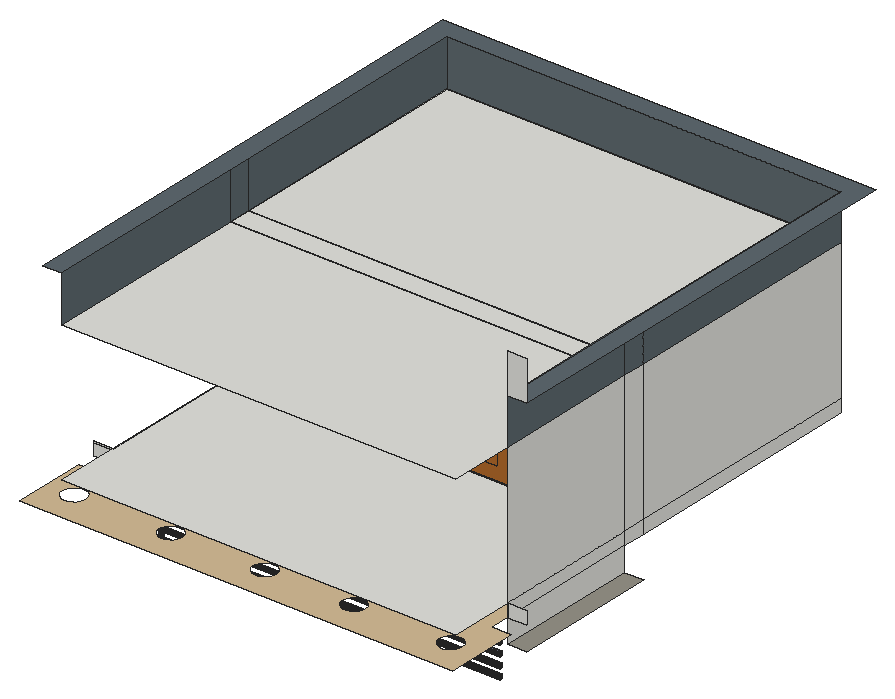
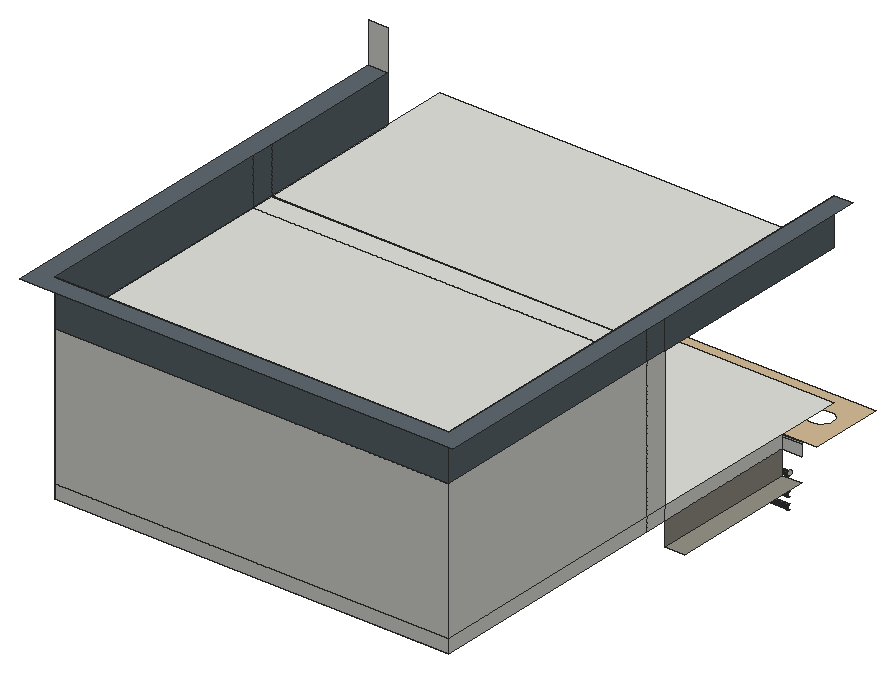
# SketchUp Ruby script. Lengths in inches.
U = 1.inch
M = Sketchup.active_model
def pt(a) = Geom::Point3d.new(a.map { |v| v * U })
def face(e, loops, mat)
  f = e.add_face(loops[0].map { |a| pt(a) })
  loops[1..].each { |l| e.add_face(l.map { |a| pt(a) }).erase! }
  f.material = f.back_material = mat if mat
  f
end
# faces: each face lists its corners as indices into pts; further lists are holes
def faces(e, pts, list, mat = nil) = list.each { |f| face(e, (f[0].is_a?(Array) ? f : [f]).map { |l| l.map { |i| pts[i] } }, mat) }
# xy, xz, yz: faces in a plane at the given z, y or x. An outline is a flat list of corners, or four numbers for a rectangle; further outlines are holes
def ring(l) = l.size == 4 ? [[l[0], l[1]], [l[2], l[1]], [l[2], l[3]], [l[0], l[3]]] : l.each_slice(2).to_a
def flat(e, list, mat, &to3) = list.each { |f| face(e, (f[0].is_a?(Array) ? f : [f]).map { |l| ring(l).map { |u, v| to3.(u, v) } }, mat) }
def xy(e, z, list, mat = nil) = flat(e, list, mat) { |x, y| [x, y, z] }
def xz(e, y, list, mat = nil) = flat(e, list, mat) { |x, z| [x, y, z] }
def yz(e, x, list, mat = nil) = flat(e, list, mat) { |y, z| [x, y, z] }
def lines(e, pts, list) = list.each { |a, b| e.add_line(pt(pts[a]), pt(pts[b])) }
# prism: a flat outline (further loops are holes) pulled along v
def prism(e, loops, v, mat = nil)
  f = face(e, loops, mat); d = Geom::Vector3d.new(v.map { |x| x * U })
  f.pushpull(f.normal.samedirection?(d) ? d.length : -d.length)
end
def box(e, o, s, mat = nil) = prism(e, [[o, [o[0] + s[0], o[1], o[2]], [o[0] + s[0], o[1] + s[1], o[2]], [o[0], o[1] + s[1], o[2]]]], [0, 0, s[2]], mat)
def at(x, y, z, deg = 0) = Geom::Transformation.translation(pt([x, y, z])) * Geom::Transformation.rotation(ORIGIN, Z_AXIS, deg.degrees)
def axes(o, x, y, z) = Geom::Transformation.new([*x, 0, *y, 0, *z, 0, *pt(o).to_a, 1])
def part(name) = M.definitions.add(name)
# library, detail: a bought-in or finely detailed component or shape, given as its bounding box
def library(name, o, s) = part(name).tap { |d| box(d.entities, o, s) }
def detail(e, o, s) = box(e.add_group.entities, o, s)
def put(e, d, t, mat = nil) = e.add_instance(d, t).tap { |i| i.material = mat if mat }
def group(e, t, mat = nil) = e.add_group.tap { |g| g.transformation = t; g.material = mat if mat }.entities
root = M.entities
M.materials.add("[Blinds Cloth Horizontal]").color = [192, 163, 85]
M.materials.add("[Formica Beige]").color = [211, 187, 149]
M.materials.add("[Formica Graystone]").color = [149, 146, 135]
M.materials.add("[Formica Laminate Dark]").color = [50, 53, 60]
M.materials.add("[Formica Speckled Grey]").color = [94, 105, 111]
M.materials.add("[Metal Steel Textured]").color = [106, 110, 123]
M.materials.add("[Wood Bamboo]").color = [177, 105, 43]
M.materials.add("[Wood Cherry Original]").color = [152, 86, 42]
xy(root,38.97,[[48.11,54.44,47.99,54.46,47.89,54.5,47.8,54.57,47.73,54.66,47.68,54.77,47.67,54.88,47.68,54.99,47.73,55.1,47.8,55.19,47.89,55.26,47.99,55.3,48.11,55.32,48.22,55.3,48.33,55.26,48.42,55.19,48.49,55.1,48.53,54.99,48.54,54.88,48.53,54.77,48.49,54.66,48.42,54.57,48.33,54.5,48.22,54.46]])
xy(root,39.16,[[51.04,54.44,50.93,54.46,50.83,54.5,50.74,54.57,50.67,54.66,50.62,54.77,50.61,54.88,50.62,54.99,50.67,55.1,50.74,55.19,50.83,55.26,50.93,55.3,51.04,55.32,51.16,55.3,51.26,55.26,51.35,55.19,51.42,55.1,51.47,54.99,51.48,54.88,51.47,54.77,51.42,54.66,51.35,54.57,51.26,54.5,51.16,54.46]])
xy(root,39.53,[[68.17,54.44,68.06,54.46,67.95,54.5,67.86,54.57,67.79,54.66,67.75,54.77,67.73,54.88,67.75,54.99,67.79,55.1,67.86,55.19,67.95,55.26,68.06,55.3,68.17,55.32,68.28,55.3,68.39,55.26,68.48,55.19,68.55,55.1,68.59,54.99,68.61,54.88,68.59,54.77,68.55,54.66,68.48,54.57,68.39,54.5,68.28,54.46]])
xy(root,39.72,[[71.42,54.44,71.31,54.46,71.2,54.5,71.11,54.57,71.04,54.66,71,54.77,70.98,54.88,71,54.99,71.04,55.1,71.11,55.19,71.2,55.26,71.31,55.3,71.42,55.32,71.53,55.3,71.64,55.26,71.73,55.19,71.8,55.1,71.84,54.99,71.86,54.88,71.84,54.77,71.8,54.66,71.73,54.57,71.64,54.5,71.53,54.46]])
xy(root,40.3,[[92.4,92.52,118.56,98]])
xy(root,46.9375,[[33.03,57.16,37.72,92.52],[133.09,57.16,137.78,92.52]],"[Formica Graystone]")
xy(root,48.59,[[48.11,54.44,48.22,54.46,48.33,54.5,48.42,54.57,48.49,54.66,48.53,54.77,48.54,54.88,48.53,54.99,48.49,55.1,48.42,55.19,48.33,55.26,48.22,55.3,48.11,55.32,47.99,55.3,47.89,55.26,47.8,55.19,47.73,55.1,47.68,54.99,47.67,54.88,47.68,54.77,47.73,54.66,47.8,54.57,47.89,54.5,47.99,54.46],[51.04,54.44,51.16,54.46,51.26,54.5,51.35,54.57,51.42,54.66,51.47,54.77,51.48,54.88,51.47,54.99,51.42,55.1,51.35,55.19,51.26,55.26,51.16,55.3,51.04,55.32,50.93,55.3,50.83,55.26,50.74,55.19,50.67,55.1,50.62,54.99,50.61,54.88,50.62,54.77,50.67,54.66,50.74,54.57,50.83,54.5,50.93,54.46],[68.17,54.44,68.28,54.46,68.39,54.5,68.48,54.57,68.55,54.66,68.59,54.77,68.61,54.88,68.59,54.99,68.55,55.1,68.48,55.19,68.39,55.26,68.28,55.3,68.17,55.32,68.06,55.3,67.95,55.26,67.86,55.19,67.79,55.1,67.75,54.99,67.73,54.88,67.75,54.77,67.79,54.66,67.86,54.57,67.95,54.5,68.06,54.46],[71.42,54.44,71.53,54.46,71.64,54.5,71.73,54.57,71.8,54.66,71.84,54.77,71.86,54.88,71.84,54.99,71.8,55.1,71.73,55.19,71.64,55.26,71.53,55.3,71.42,55.32,71.31,55.3,71.2,55.26,71.11,55.19,71.04,55.1,71,54.99,70.98,54.88,71,54.77,71.04,54.66,71.11,54.57,71.2,54.5,71.31,54.46]])
xy(root,52.6875,[[37.72,92.52,133.09,98],[37.72,98,133.09,158.08]])
xy(root,52.6875,[[[33.03,34.66,33.03,52.46,91.56,52.46,91.56,57.16,37.72,57.16,37.72,92.52,133.09,92.52,133.09,52.46,137.78,52.46,137.78,34.66],[39.58,40.0625,40.32,40.16,41.01,40.45,41.61,40.9,42.07,41.5,42.35,42.19,42.45,42.9375,42.35,43.68,42.07,44.375,41.61,44.97,41.01,45.43,40.32,45.71,39.58,45.8125,38.83,45.71,38.14,45.43,37.54,44.97,37.09,44.375,36.8,43.68,36.7,42.9375,36.8,42.19,37.09,41.5,37.54,40.9,38.14,40.45,38.83,40.16],[130.7,40.0625,131.44,40.16,132.14,40.45,132.73,40.9,133.19,41.5,133.48,42.19,133.58,42.9375,133.48,43.68,133.19,44.375,132.73,44.97,132.14,45.43,131.44,45.71,130.7,45.8125,129.96,45.71,129.26,45.43,128.67,44.97,128.21,44.375,127.92,43.68,127.83,42.9375,127.92,42.19,128.21,41.5,128.67,40.9,129.26,40.45,129.96,40.16],[63.01,40.0625,63.76,40.16,64.45,40.45,65.05,40.9,65.5,41.5,65.79,42.19,65.89,42.9375,65.79,43.68,65.5,44.375,65.05,44.97,64.45,45.43,63.76,45.71,63.01,45.8125,62.27,45.71,61.58,45.43,60.98,44.97,60.52,44.375,60.24,43.68,60.14,42.9375,60.24,42.19,60.52,41.5,60.98,40.9,61.58,40.45,62.27,40.16],[107.2,40.0625,107.94,40.16,108.64,40.45,109.23,40.9,109.69,41.5,109.98,42.19,110.08,42.9375,109.98,43.68,109.69,44.375,109.23,44.97,108.64,45.43,107.94,45.71,107.2,45.8125,106.46,45.71,105.76,45.43,105.17,44.97,104.71,44.375,104.42,43.68,104.33,42.9375,104.42,42.19,104.71,41.5,105.17,40.9,105.76,40.45,106.46,40.16],[85.76,40.0625,86.51,40.16,87.2,40.45,87.8,40.9,88.25,41.5,88.54,42.19,88.64,42.9375,88.54,43.68,88.25,44.375,87.8,44.97,87.2,45.43,86.51,45.71,85.76,45.8125,85.02,45.71,84.33,45.43,83.73,44.97,83.27,44.375,82.99,43.68,82.89,42.9375,82.99,42.19,83.27,41.5,83.73,40.9,84.33,40.45,85.02,40.16]]],"[Formica Beige]")
xy(root,55.875,[[37.72,41.5,133.09,92.52],[37.72,92.52,133.09,98],[37.72,98,133.09,158.08]])
xy(root,89.5625,[[37.72,41.5,133.09,92.52],[37.72,92.52,133.09,98],[37.72,98,133.09,158.08]])
xy(root,100.8125,[[33.03,41.5,37.72,41.5,37.72,158.08,133.09,158.08,133.09,57.16,137.78,57.16,137.78,162.77,33.03,162.77]],"[Formica Speckled Grey]")
xz(root,57.16,[[37.72,48.59,82.62,52.6875],[33.03,52.6875,37.72,55.4375],[133.09,52.6875,137.78,55.875],[33.03,55.4375,37.72,55.875],[133.09,100.8125,137.78,110.5625]])
xz(root,92.52,[[37.72,52.6875,88.58,55.875],[88.58,52.6875,122.39,55.875],[122.39,52.6875,133.09,55.875],[[37.72,55.875,86.42,55.875,86.42,84.9,105.48,84.9,105.48,55.875,133.09,55.875,133.09,89.5625,37.72,89.5625],[50.84,62.65,75.9,85.28]]])
xz(root,92.52,[[52.83,64.65,60.27,83.28],[62.42,64.65,73.9,83.28]],"[Blinds Cloth Horizontal]")
xz(root,92.52,[[[86.42,55.875,105.48,84.9],[89.56,59.01,102.35,81.77]],[89.56,59.01,102.35,81.77]],"[Wood Bamboo]")
xz(root,92.52,[[[50.84,62.65,75.9,85.28],[52.83,64.65,73.9,83.28]],[60.27,64.65,62.42,83.28]],"[Wood Cherry Original]")
xz(root,98,[[37.72,52.6875,133.09,55.875],[37.72,55.875,133.09,89.5625]])
xz(root,158.08,[[37.72,52.6875,133.09,55.875],[37.72,55.875,133.09,89.5625]])
xz(root,158.08,[[37.72,89.5625,133.09,100.8125]],"[Formica Speckled Grey]")
yz(root,37.72,[[54.84,45.92,54.69,45.94,54.56,46,54.44,46.09,54.35,46.2,54.3,46.34,54.28,46.48,54.3,46.63,54.35,46.77,54.44,46.88,54.56,46.97,54.69,47.03,54.84,47.05,54.99,47.03,55.12,46.97,55.24,46.88,55.33,46.77,55.38,46.63,55.4,46.48,55.38,46.34,55.33,46.2,55.24,46.09,55.12,46,54.99,45.94],[57.16,52.6875,92.52,55.875],[92.52,52.6875,98,55.875],[98,52.6875,158.08,55.875],[92.52,55.875,98,89.5625],
  [98,55.875,158.08,89.5625]])
yz(root,37.72,[[57.16,46.9375,92.52,52.6875]],"[Formica Graystone]")
yz(root,37.72,[[41.5,89.5625,92.52,100.8125],[92.52,89.5625,98,100.8125],[98,89.5625,158.08,100.8125]],"[Formica Speckled Grey]")
yz(root,91.56,[[55.04,40.18,54.9,40.2,54.76,40.26,54.64,40.35,54.55,40.46,54.5,40.6,54.48,40.75,54.5,40.89,54.55,41.03,54.64,41.14,54.76,41.23,54.9,41.29,55.04,41.31,55.1875,41.29,55.32,41.23,55.4375,41.14,55.53,41.03,55.58,40.89,55.6,40.75,55.58,40.6,55.53,40.46,55.4375,40.35,55.32,40.26,55.1875,40.2],[55.04,42.56,54.9,42.58,54.76,42.63,54.64,42.72,54.55,42.84,54.5,42.98,54.48,43.12,54.5,43.27,54.55,43.4,54.64,43.52,54.76,43.61,54.9,43.66,55.04,43.68,55.1875,43.66,55.32,43.61,55.4375,43.52,55.53,43.4,55.58,43.27,55.6,43.12,55.58,42.98,55.53,42.84,55.4375,42.72,55.32,42.63,55.1875,42.58],[55.04,45.18,54.9,45.2,54.76,45.26,54.64,45.35,54.55,45.46,54.5,45.6,54.48,45.75,54.5,45.89,54.55,46.03,54.64,46.14,54.76,46.23,54.9,46.29,55.04,46.31,55.1875,46.29,55.32,46.23,55.4375,46.14,55.53,46.03,55.58,45.89,55.6,45.75,55.58,45.6,55.53,45.46,55.4375,45.35,55.32,45.26,55.1875,45.2],[55.04,47.68,54.9,47.7,54.76,47.76,54.64,47.85,54.55,47.96,54.5,48.1,54.48,48.25,54.5,48.39,54.55,48.53,54.64,48.64,54.76,48.73,54.9,48.79,55.04,48.81,55.1875,48.79,55.32,48.73,55.4375,48.64,55.53,48.53,55.58,48.39,55.6,48.25,55.58,48.1,55.53,47.96,55.4375,47.85,55.32,47.76,55.1875,47.7]])
yz(root,133.09,[[57.16,46.9375,92.52,52.6875],[57.16,52.6875,92.52,55.875],[92.52,52.6875,98,55.875],[98,52.6875,158.08,55.875],[57.16,55.875,92.52,89.5625],
  [92.52,55.875,98,89.5625],[98,55.875,158.08,89.5625]])
yz(root,133.09,[[57.16,89.5625,92.52,100.8125],[92.52,89.5625,98,100.8125],[98,89.5625,158.08,100.8125]],"[Formica Speckled Grey]")
p = [[37.72,54.84,38.61],[37.72,54.99,38.63],[82.62,54.99,38.63],[82.62,54.84,38.61],[37.72,55.12,38.68],[82.62,55.12,38.68],
  [37.72,55.24,38.77],[82.62,55.24,38.77],[37.72,55.33,38.89],[82.62,55.33,38.89],[37.72,55.38,39.03],[82.62,55.38,39.03],
  [47.67,54.88,48.59],[47.68,54.99,48.59],[47.68,54.99,38.97],[47.67,54.88,38.97],[48.53,54.99,48.59],[48.54,54.88,48.59],
  [48.54,54.88,38.97],[48.53,54.99,38.97],[47.73,55.1,48.59],[47.73,55.1,38.97],[48.49,55.1,48.59],[48.49,55.1,38.97],
  [47.8,55.19,48.59],[47.8,55.19,38.97],[48.42,55.19,48.59],[48.42,55.19,38.97],[47.89,55.26,48.59],[47.89,55.26,38.97],
  [48.33,55.26,48.59],[48.33,55.26,38.97],[47.99,55.3,48.59],[47.99,55.3,38.97],[48.11,55.32,48.59],[48.11,55.32,38.97],
  [48.22,55.3,48.59],[48.22,55.3,38.97],[37.72,55.4,39.17],[82.62,55.4,39.17],[50.61,54.88,48.59],[50.62,54.99,48.59],
  [50.62,54.99,39.16],[50.61,54.88,39.16],[51.47,54.99,48.59],[51.48,54.88,48.59],[51.48,54.88,39.16],[51.47,54.99,39.16],
  [50.67,55.1,48.59],[50.67,55.1,39.16],[51.42,55.1,48.59],[51.42,55.1,39.16],[50.74,55.19,48.59],[50.74,55.19,39.16],
  [51.35,55.19,48.59],[51.35,55.19,39.16],[50.83,55.26,48.59],[50.83,55.26,39.16],[51.26,55.26,48.59],[51.26,55.26,39.16],
  [50.93,55.3,48.59],[50.93,55.3,39.16],[51.04,55.32,48.59],[51.04,55.32,39.16],[51.16,55.3,48.59],[51.16,55.3,39.16],
  [37.72,55.38,39.32],[82.62,55.38,39.32],[37.72,55.33,39.45],[82.62,55.33,39.45],[67.73,54.88,48.59],[67.75,54.99,48.59],
  [67.75,54.99,39.53],[67.73,54.88,39.53],[68.59,54.99,48.59],[68.61,54.88,48.59],[68.61,54.88,39.53],[68.59,54.99,39.53],
  [67.79,55.1,48.59],[67.79,55.1,39.53],[68.55,55.1,48.59],[68.55,55.1,39.53],[67.86,55.19,48.59],[67.86,55.19,39.53],
  [68.48,55.19,48.59],[68.48,55.19,39.53],[37.72,55.24,39.57],[82.62,55.24,39.57],[67.95,55.26,48.59],[67.95,55.26,39.53],
  [68.39,55.26,48.59],[68.39,55.26,39.53],[68.06,55.3,48.59],[68.06,55.3,39.53],[68.17,55.32,48.59],[68.17,55.32,39.53],
  [68.28,55.3,48.59],[68.28,55.3,39.53],[37.72,55.12,39.66],[82.62,55.12,39.66],[37.72,54.99,39.72],[37.72,54.84,39.73],
  [82.62,54.84,39.73],[82.62,54.99,39.72],[70.98,54.88,48.59],[71,54.99,48.59],[71,54.99,39.72],[70.98,54.88,39.72],
  [71.84,54.99,48.59],[71.86,54.88,48.59],[71.86,54.88,39.72],[71.84,54.99,39.72],[71.04,55.1,48.59],[71.04,55.1,39.72],
  [71.8,55.1,48.59],[71.8,55.1,39.72],[71.11,55.19,48.59],[71.11,55.19,39.72],[71.73,55.19,48.59],[71.73,55.19,39.72],
  [71.2,55.26,48.59],[71.2,55.26,39.72],[71.64,55.26,48.59],[71.64,55.26,39.72],[71.31,55.3,48.59],[71.31,55.3,39.72],
  [71.42,55.32,48.59],[71.42,55.32,39.72],[71.53,55.3,48.59],[71.53,55.3,39.72],[91.56,54.9,40.2],[91.56,55.04,40.18],
  [133.09,55.04,40.18],[133.09,54.9,40.2],[91.56,55.1875,40.2],[133.09,55.1875,40.2],[91.56,55.32,40.26],[133.09,55.32,40.26],
  [91.56,55.4375,40.35],[133.09,55.4375,40.35],[91.56,55.53,40.46],[133.09,55.53,40.46],[91.56,55.58,40.6],[133.09,55.58,40.6],
  [91.56,55.6,40.75],[133.09,55.6,40.75],[91.56,55.58,40.89],[133.09,55.58,40.89],[91.56,55.53,41.03],[133.09,55.53,41.03],
  [91.56,55.4375,41.14],[133.09,55.4375,41.14],[91.56,55.32,41.23],[133.09,55.32,41.23],[91.56,55.1875,41.29],[133.09,55.1875,41.29],
  [91.56,55.04,41.31],[91.56,54.9,41.29],[133.09,54.9,41.29],[133.09,55.04,41.31],[37.72,54.84,41.36],[37.72,54.99,41.38],
  [82.62,54.99,41.38],[82.62,54.84,41.36],[37.72,55.12,41.43],[82.62,55.12,41.43],[37.72,55.24,41.52],[82.62,55.24,41.52],
  [37.72,55.33,41.64],[82.62,55.33,41.64],[37.72,55.38,41.78],[82.62,55.38,41.78],[37.72,55.4,41.92],[82.62,55.4,41.92],
  [37.72,55.38,42.07],[82.62,55.38,42.07],[37.72,55.33,42.2],[82.62,55.33,42.2],[37.72,55.24,42.32],[82.62,55.24,42.32],
  [37.72,55.12,42.41],[82.62,55.12,42.41],[37.72,54.99,42.47],[82.62,54.99,42.47],[37.72,54.84,42.48],[82.62,54.84,42.48],
  [91.56,54.9,42.58],[91.56,55.04,42.56],[133.09,55.04,42.56],[133.09,54.9,42.58],[91.56,55.1875,42.58],[133.09,55.1875,42.58],
  [91.56,55.32,42.63],[133.09,55.32,42.63],[91.56,55.4375,42.72],[133.09,55.4375,42.72],[91.56,55.53,42.84],[133.09,55.53,42.84],
  [91.56,55.58,42.98],[133.09,55.58,42.98],[91.56,55.6,43.12],[133.09,55.6,43.12],[91.56,55.58,43.27],[133.09,55.58,43.27],
  [91.56,55.53,43.4],[133.09,55.53,43.4],[91.56,55.4375,43.52],[133.09,55.4375,43.52],[91.56,55.32,43.61],[133.09,55.32,43.61],
  [91.56,55.1875,43.66],[133.09,55.1875,43.66],[37.72,54.84,43.67],[37.72,54.99,43.69],[82.62,54.99,43.69],[82.62,54.84,43.67],
  [91.56,55.04,43.68],[91.56,54.9,43.66],[133.09,54.9,43.66],[133.09,55.04,43.68],[37.72,55.12,43.75],[82.62,55.12,43.75],
  [37.72,55.24,43.84],[82.62,55.24,43.84],[37.72,55.33,43.95],[82.62,55.33,43.95],[37.72,55.38,44.09],[82.62,55.38,44.09],
  [37.72,55.4,44.23],[82.62,55.4,44.23],[37.72,55.38,44.38],[82.62,55.38,44.38],[37.72,55.33,44.52],[82.62,55.33,44.52],
  [37.72,55.24,44.63],[82.62,55.24,44.63],[37.72,55.12,44.72],[82.62,55.12,44.72],[37.72,54.99,44.78],[82.62,54.99,44.78],
  [37.72,54.84,44.8],[82.62,54.84,44.8],[91.56,54.9,45.2],[91.56,55.04,45.18],[133.09,55.04,45.18],[133.09,54.9,45.2],
  [91.56,55.1875,45.2],[133.09,55.1875,45.2],[91.56,55.32,45.26],[133.09,55.32,45.26],[91.56,55.4375,45.35],[133.09,55.4375,45.35],
  [91.56,55.53,45.46],[133.09,55.53,45.46],[91.56,55.58,45.6],[133.09,55.58,45.6],[91.56,55.6,45.75],[133.09,55.6,45.75],
  [91.56,55.58,45.89],[133.09,55.58,45.89],[37.72,54.84,45.92],[37.72,54.99,45.94],[82.62,54.99,45.94],[82.62,54.84,45.92],
  [37.72,55.12,46],[82.62,55.12,46],[91.56,55.53,46.03],[133.09,55.53,46.03],[37.72,55.24,46.09],[82.62,55.24,46.09],
  [91.56,55.4375,46.14],[133.09,55.4375,46.14],[37.72,55.33,46.2],[82.62,55.33,46.2],[91.56,55.32,46.23],[133.09,55.32,46.23],
  [91.56,55.1875,46.29],[133.09,55.1875,46.29],[37.72,55.38,46.34],[82.62,55.38,46.34],[91.56,55.04,46.31],[91.56,54.9,46.29],
  [133.09,54.9,46.29],[133.09,55.04,46.31],[37.72,55.4,46.48],[82.62,55.4,46.48],[37.72,55.38,46.63],[82.62,55.38,46.63],
  [37.72,55.33,46.77],[82.62,55.33,46.77],[37.72,55.24,46.88],[82.62,55.24,46.88],[37.72,55.12,46.97],[82.62,55.12,46.97],
  [37.72,54.99,47.03],[37.72,54.84,47.05],[82.62,54.84,47.05],[82.62,54.99,47.03],[91.56,54.9,47.7],[91.56,55.04,47.68],
  [133.09,55.04,47.68],[133.09,54.9,47.7],[91.56,55.1875,47.7],[133.09,55.1875,47.7],[91.56,55.32,47.76],[133.09,55.32,47.76],
  [91.56,55.4375,47.85],[133.09,55.4375,47.85],[91.56,55.53,47.96],[133.09,55.53,47.96],[91.56,55.58,48.1],[133.09,55.58,48.1],
  [91.56,55.6,48.25],[133.09,55.6,48.25],[91.56,55.58,48.39],[133.09,55.58,48.39],[91.56,55.53,48.53],[133.09,55.53,48.53],
  [91.56,55.4375,48.64],[133.09,55.4375,48.64],[91.56,55.32,48.73],[133.09,55.32,48.73],[91.56,55.1875,48.79],[133.09,55.1875,48.79],
  [91.56,55.04,48.81],[91.56,54.9,48.79],[133.09,54.9,48.79],[133.09,55.04,48.81]]
faces(root,p,[[0,1,2,3],[1,4,5,2],[4,6,7,5],[6,8,9,7],[8,10,11,9],[10,38,39,11],[38,66,67,39],[66,68,69,67],
  [68,86,87,69],[86,98,99,87],[100,101,102,103],[98,100,103,99],[130,131,132,133],[131,134,135,132],[134,136,137,135],[136,138,139,137],
  [138,140,141,139],[140,142,143,141],[142,144,145,143],[144,146,147,145],[146,148,149,147],[148,150,151,149],[150,152,153,151],[152,154,155,153],
  [156,157,158,159],[154,156,159,155],[160,161,162,163],[161,164,165,162],[164,166,167,165],[166,168,169,167],[168,170,171,169],[170,172,173,171],
  [172,174,175,173],[174,176,177,175],[176,178,179,177],[178,180,181,179],[180,182,183,181],[182,184,185,183],[186,187,188,189],[187,190,191,188],
  [190,192,193,191],[192,194,195,193],[194,196,197,195],[196,198,199,197],[198,200,201,199],[200,202,203,201],[202,204,205,203],[204,206,207,205],
  [206,208,209,207],[208,210,211,209],[212,213,214,215],[216,217,218,219],[213,220,221,214],[210,216,219,211],[220,222,223,221],[222,224,225,223],
  [224,226,227,225],[226,228,229,227],[228,230,231,229],[230,232,233,231],[232,234,235,233],[234,236,237,235],[236,238,239,237],[238,240,241,239],
  [242,243,244,245],[243,246,247,244],[246,248,249,247],[248,250,251,249],[250,252,253,251],[252,254,255,253],[254,256,257,255],[256,258,259,257],
  [260,261,262,263],[261,264,265,262],[258,266,267,259],[264,268,269,265],[266,270,271,267],[268,272,273,269],[270,274,275,271],[274,276,277,275],
  [272,278,279,273],[280,281,282,283],[276,280,283,277],[278,284,285,279],[284,286,287,285],[286,288,289,287],[288,290,291,289],[290,292,293,291],
  [294,295,296,297],[292,294,297,293],[298,299,300,301],[299,302,303,300],[302,304,305,303],[304,306,307,305],[306,308,309,307],[308,310,311,309],
  [310,312,313,311],[312,314,315,313],[314,316,317,315],[316,318,319,317],[318,320,321,319],[320,322,323,321],[324,325,326,327],[322,324,327,323]],"[Metal Steel Textured]")
faces(root,p,[[12,13,14,15],[16,17,18,19],[13,20,21,14],[22,16,19,23],[20,24,25,21],[26,22,23,27],[24,28,29,25],[30,26,27,31],
  [28,32,33,29],[32,34,35,33],[34,36,37,35],[36,30,31,37],[40,41,42,43],[44,45,46,47],[41,48,49,42],[50,44,47,51],
  [48,52,53,49],[54,50,51,55],[52,56,57,53],[58,54,55,59],[56,60,61,57],[60,62,63,61],[62,64,65,63],[64,58,59,65],
  [70,71,72,73],[74,75,76,77],[71,78,79,72],[80,74,77,81],[78,82,83,79],[84,80,81,85],[82,88,89,83],[90,84,85,91],
  [88,92,93,89],[92,94,95,93],[94,96,97,95],[96,90,91,97],[104,105,106,107],[108,109,110,111],[105,112,113,106],[114,108,111,115],
  [112,116,117,113],[118,114,115,119],[116,120,121,117],[122,118,119,123],[120,124,125,121],[124,126,127,125],[126,128,129,127],[128,122,123,129]],"[Formica Laminate Dark]")
